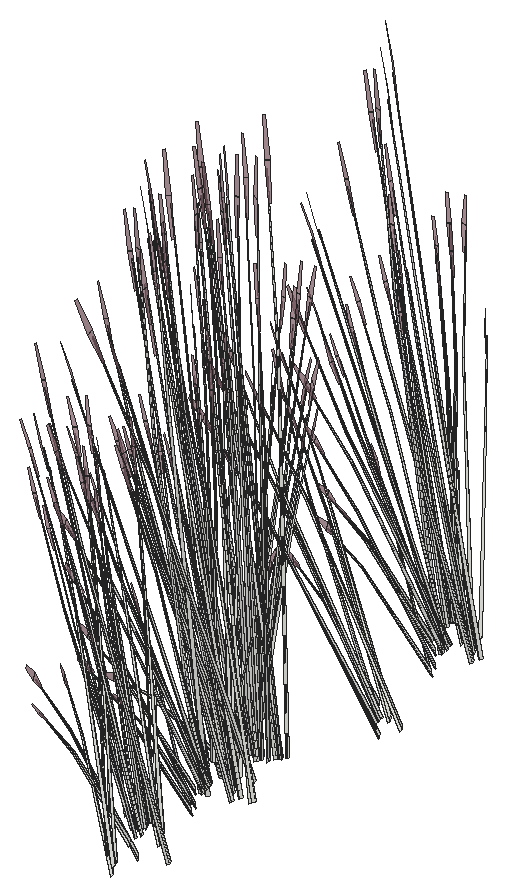
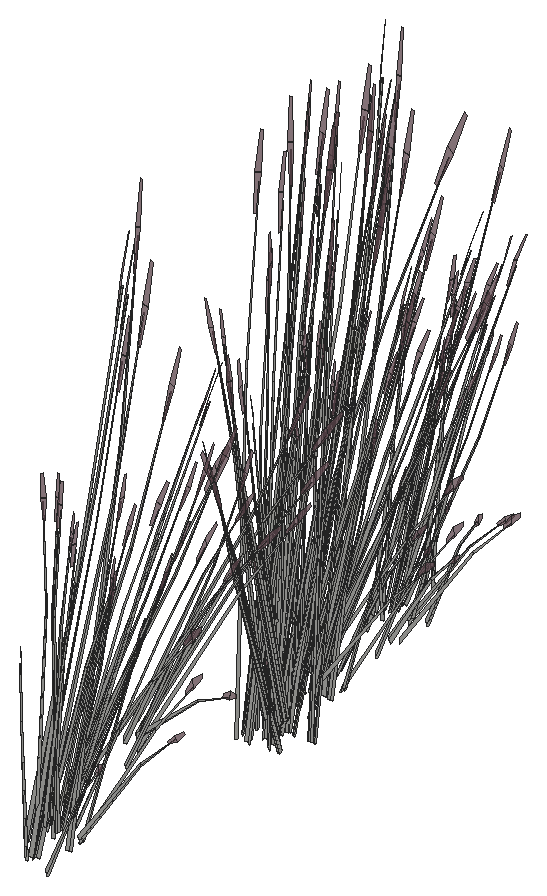
# SketchUp Ruby script. Lengths in inches.
U = 1.inch
M = Sketchup.active_model
def pt(a) = Geom::Point3d.new(a.map { |v| v * U })
def face(e, loops, mat)
  f = e.add_face(loops[0].map { |a| pt(a) })
  loops[1..].each { |l| e.add_face(l.map { |a| pt(a) }).erase! }
  f.material = f.back_material = mat if mat
  f
end
# faces: each face lists its corners as indices into pts; further lists are holes
def faces(e, pts, list, mat = nil) = list.each { |f| face(e, (f[0].is_a?(Array) ? f : [f]).map { |l| l.map { |i| pts[i] } }, mat) }
# xy, xz, yz: faces in a plane at the given z, y or x. An outline is a flat list of corners, or four numbers for a rectangle; further outlines are holes
def ring(l) = l.size == 4 ? [[l[0], l[1]], [l[2], l[1]], [l[2], l[3]], [l[0], l[3]]] : l.each_slice(2).to_a
def flat(e, list, mat, &to3) = list.each { |f| face(e, (f[0].is_a?(Array) ? f : [f]).map { |l| ring(l).map { |u, v| to3.(u, v) } }, mat) }
def xy(e, z, list, mat = nil) = flat(e, list, mat) { |x, y| [x, y, z] }
def xz(e, y, list, mat = nil) = flat(e, list, mat) { |x, z| [x, y, z] }
def yz(e, x, list, mat = nil) = flat(e, list, mat) { |y, z| [x, y, z] }
def lines(e, pts, list) = list.each { |a, b| e.add_line(pt(pts[a]), pt(pts[b])) }
# prism: a flat outline (further loops are holes) pulled along v
def prism(e, loops, v, mat = nil)
  f = face(e, loops, mat); d = Geom::Vector3d.new(v.map { |x| x * U })
  f.pushpull(f.normal.samedirection?(d) ? d.length : -d.length)
end
def box(e, o, s, mat = nil) = prism(e, [[o, [o[0] + s[0], o[1], o[2]], [o[0] + s[0], o[1] + s[1], o[2]], [o[0], o[1] + s[1], o[2]]]], [0, 0, s[2]], mat)
def at(x, y, z, deg = 0) = Geom::Transformation.translation(pt([x, y, z])) * Geom::Transformation.rotation(ORIGIN, Z_AXIS, deg.degrees)
def axes(o, x, y, z) = Geom::Transformation.new([*x, 0, *y, 0, *z, 0, *pt(o).to_a, 1])
def part(name) = M.definitions.add(name)
# library, detail: a bought-in or finely detailed component or shape, given as its bounding box
def library(name, o, s) = part(name).tap { |d| box(d.entities, o, s) }
def detail(e, o, s) = box(e.add_group.entities, o, s)
def put(e, d, t, mat = nil) = e.add_instance(d, t).tap { |i| i.material = mat if mat }
def group(e, t, mat = nil) = e.add_group.tap { |g| g.transformation = t; g.material = mat if mat }.entities
root = M.entities
M.materials.add("LightPink_Translucent").color = [144, 107, 117]
M.materials["LightPink_Translucent"].alpha = 0.75
c1 = part("blade")
p = [[2.15,0.21,22],[0,0.17,0],[0.09,0.45,0],[2.18,0.31,22],[2.29,0.31,22],[0.38,0.45,0],
  [2.48,0.24,33],[2.49,0.24,33],[2.48,0.22,33]]
faces(c1.entities,p,[[0,1,2,3],[4,5,2,3],[6,3,4,7],[8,0,3,6]])
c2 = part("seeds")
p = [[0.3,-0.1,1.38],[-0.01,-0.03,1.59],[-0.01,-0.03,0.03],[0.14,-0.07,-0.07],[0.29,-0.03,3],[0.15,0.01,3.11]]
faces(c2.entities,p,[[0,1,2,3],[1,0,4,5]],"LightPink_Translucent")
c3 = part("blade with seeds")
put(c3.entities,c1,at(0,0,0))
put(c3.entities,c2,axes([2.4,0.25,30.99],[1.5799,-0.05474,1.17369],[-0.12525,1.92788,0.29478],[-0.07173,-0.02425,1.56792]))
put(root,c3,axes([287.68,481.24,4.73],[-0.61415,-0.2744,0.0643],[0.35756,-0.39076,0.50621],[-0.1969,0.12633,0.77189]))
put(root,c3,axes([287.0625,487.16,2.21],[-0.53742,-0.54764,-0.44739],[0.81403,-0.38564,0.21531],[-0.17391,-0.06776,1.43643]))
put(root,c3,axes([288.45,511.57,4.73],[-0.32857,-0.44488,0.0643],[0.59916,-0.21775,0.50621],[-0.26412,0.04296,0.77189]))
put(root,c3,axes([289.96,512.8,3.875],[0.22344,-0.20048,1.71376],[0.56419,0.54113,0.13857],[-0.38697,0.24643,0.73262]))
put(root,c3,axes([288.62,513.33,4.53],[-0.77872,0.09325,-0.35414],[-0.20563,-0.53305,0.4572],[-0.22316,0.14318,0.87481]))
put(root,c3,axes([285.54,488.6,5.34],[-0.02328,0.60353,-0.7886],[-0.98022,-0.04053,0.09517],[-0.10344,0.25568,1.11556]))
put(root,c3,axes([285.52,490.3,2.77],[-0.02315,-0.38796,1.1486],[0.57853,0.27671,0.84392],[-0.11378,0.18492,0.25299]))
put(root,c3,axes([286.33,483.67,5.09],[0.99656,-0.1677,0.53763],[0.17295,0.65785,0.4433],[-0.23438,-0.19388,1.11249]))
put(root,c3,axes([290.03,468.16,4.53],[-0.74348,-0.18202,-0.35414],[0.21685,-0.53102,0.4572],[-0.29933,0.04869,0.87481]))
put(root,c3,axes([288.19,514.91,1.49],[0.12,0.06519,1.76342],[0.20347,0.60397,-0.26939],[-0.26596,0.12879,0.30037]))
put(root,c3,axes([288.93,481.44,3.875],[0.16657,-0.22426,1.71376],[0.69879,0.4641,0.13857],[-0.31524,0.28926,0.73262]))
put(root,c3,axes([288.21,487.55,2.21],[-0.97146,0.04028,-0.44739],[-0.08785,-0.66859,0.21531],[-0.17391,0.06776,1.43643]))
put(root,c3,axes([288.02,511.36,2.77],[0.57115,-0.04669,1.1486],[-0.36229,0.41137,0.84392],[-0.28224,-0.06171,0.25299]))
put(root,c3,axes([288.26,479.88,5.05],[0.74348,0.18202,0.35414],[-0.21685,0.53102,-0.4572],[-0.29933,0.04869,0.87481]))
put(root,c3,axes([286.5625,483.81,4.73],[0.4066,-0.41448,0.0643],[0.57901,0.24131,0.50621],[-0.18719,-0.13288,0.77189]))
put(root,c3,axes([288.72,513.21,4.73],[-0.22187,-0.60049,0.48003],[0.87033,-0.10422,0.3958],[-0.25651,0.14123,0.9933]))
put(root,c3,axes([287.9375,469.14,4.71],[0.11417,0.0175,1.77383],[0.35319,0.57649,-0.16761],[-0.23371,0.15131,0.31391]))
put(root,c3,axes([290.54,468.43,4.68],[-0.24236,0.59349,-0.51099],[-0.83094,-0.20343,-0.3958],[-0.33455,0.05442,0.97773]))
put(root,c3,axes([286.35,488.67,2.48],[0.83726,0.32623,0.49651],[-0.50045,0.58498,0],[-0.19069,-0.0743,1.57504]))
put(root,c3,axes([288.39,481.53,4.68],[0.22982,0.59576,-0.51099],[-0.87033,0.10422,-0.3958],[-0.24941,0.16002,0.97773]))
put(root,c3,axes([285.21,489.45,3.36],[0.01966,-0.33682,1.54345],[0.88405,0.17791,0.21329],[-0.0766,0.35897,0.72882]))
put(root,c3,axes([289.17,510.22,5.09],[0.7388,-0.48151,0.53763],[0.63717,0.51135,0.4433],[-0.34662,-0.08882,1.11249]))
put(root,c3,axes([288.64,478.36,4.73],[0.04505,-0.49615,0.0643],[0.68022,0.0136,0.50621],[-0.26056,-0.05192,0.77189]))
put(root,c3,axes([287.03,482.6,4.72],[-0.02224,0.12912,1.74944],[0.63107,0.44917,-0.27667],[-0.16521,0.21241,0.14031]))
put(root,c3,axes([287.14,487.47,2.4375],[0.23711,-0.77313,-0.23429],[1.12425,0.13477,0.51271],[-0.19645,-0.10677,1.5644]))
put(root,c3,axes([288.54,513.1,4.73],[-0.61415,-0.2744,0.0643],[0.35756,-0.39076,0.50621],[-0.1969,0.12633,0.77189]))
put(root,c3,axes([290.12,468.39,1.49],[0.02269,0.10283,1.76342],[-0.45738,0.53699,-0.26939],[-0.32488,-0.02707,0.30037]))
put(root,c3,axes([290.5625,481.11,2.06],[-0.9306,-0.10697,-0.62353],[0.19638,-0.65984,-0.16365],[-0.27771,-0.07995,1.37633]))
put(root,c3,axes([290.73,477.51,5.43],[-0.59706,0.6255,-0.13619],[-0.86465,-0.36036,-0.75594],[-0.30056,-0.17672,1.14864]))
put(root,c3,axes([287.55,487.65,2.62],[-0.17258,0.58229,0.1448],[-0.84319,-0.10108,-0.41347],[-0.15345,-0.05979,1.26744]))
put(root,c3,axes([289.1,478.74,5.05],[0.50902,0.40851,0.35414],[-0.58122,0.38671,-0.4572],[-0.29531,-0.05884,0.87481]))
put(root,c3,axes([287.45,482.58,4.72],[-0.13683,-0.09148,1.74944],[-0.91315,0.058,-0.27667],[-0.14574,-0.2188,0.14031]))
put(root,c3,axes([289.23,489.27,2.02],[-0.83726,0.32623,-0.49651],[-0.50045,-0.58498,0],[-0.19069,0.0743,1.57504]))
put(root,c3,axes([289.79,513.3,3.875],[0.16657,-0.22426,1.71376],[0.69879,0.4641,0.13857],[-0.31524,0.28926,0.73262]))
put(root,c3,axes([284.27,486.02,2.02],[0,-0.65246,-0.49651],[1.00089,0,0],[0,-0.1486,1.57504]))
put(root,c3,axes([290.47,478.01,4.98],[-0.76283,-0.31537,-0.71045],[0.54213,-0.55263,0.08574],[-0.27638,-0.1883,1.00501]))
put(root,c3,axes([284.7,486.63,2.48],[0,0.65246,0.49651],[-1.00089,0,0],[0,-0.1486,1.57504]))
put(root,c3,axes([289.28,489.1,2.19],[-0.55235,-0.65609,-0.05142],[0.93577,-0.36461,0.51607],[-0.23059,0.06247,1.6363]))
put(root,c3,axes([290.11,478.03,4.68],[-0.88277,0.1551,-0.51099],[-0.15442,-0.58737,-0.3958],[-0.23711,-0.16832,0.97773]))
put(root,c3,axes([288.89,470.97,2.77],[0.37283,-0.29571,1.1486],[0.14711,0.46813,0.84392],[-0.26943,0.08382,0.25299]))
put(root,c3,axes([293.77,496.78,3.875],[0.37107,-0.01478,1.71376],[-0.24616,0.64047,0.13857],[-0.5288,-0.03961,0.73262]))
put(root,c3,axes([289.125,511.74,5.05],[0.74348,0.18202,0.35414],[-0.21685,0.53102,-0.4572],[-0.29933,0.04869,0.87481]))
put(root,c3,axes([285.74,488.8,5],[0.64041,0.4384,-0.5672],[-0.67652,0.38394,-0.43934],[-0.09744,0.22274,1.08528]))
put(root,c3,axes([289.34,482.35,2.02],[-0.83726,-0.32623,-0.49651],[0.50045,-0.58498,0],[-0.19069,-0.0743,1.57504]))
put(root,c3,axes([290.2,468.09,4.73],[0.25275,-0.59491,0.48003],[0.83094,0.20343,0.3958],[-0.32677,0.03575,0.9933]))
put(root,c3,axes([289.03,489.02,2.03],[-0.83462,-0.16144,-0.30978],[0.21015,-0.56852,0.30978],[-0.16826,0.06556,1.38974]))
put(root,c3,axes([288.98,477.49,1.49],[-0.08666,0.08595,1.76342],[-0.87574,0.18531,-0.26939],[-0.21156,-0.16858,0.30037]))
put(root,c3,axes([287.98,481.11,5.03],[0.82753,0.35977,-0.1216],[-0.47675,0.52101,-0.67495],[-0.2338,0.18111,1.02557]))
put(root,c3,axes([285.45,488.48,5.05],[0.60531,-0.34352,0.35414],[0.573,0.39225,-0.4572],[-0.08718,0.19929,0.87481]))
put(root,c3,axes([290.5,467.92,5.03],[0.45012,0.59081,-0.1216],[-0.79888,0.29033,-0.67495],[-0.33665,0.07795,1.02557]))
put(root,c3,axes([289.26,513.39,4.68],[0.22982,0.59576,-0.51099],[-0.87033,0.10422,-0.3958],[-0.24941,0.16002,0.97773]))
put(root,c3,axes([291.51,466.69,5.03],[-0.0479,0.66354,-0.1216],[-0.90696,-0.01814,-0.67495],[-0.3493,-0.04609,1.02557]))
put(root,c3,axes([286.89,486.78,2.67],[-1.00749,-0.31132,-0.29095],[0.48511,-0.65709,-0.50002],[-0.03166,-0.16133,1.59708]))
put(root,c3,axes([289.51,486.59,2.84],[-0.02444,-0.61432,1.41272],[1.10603,0.15924,0.59816],[-0.26159,0.33615,1.3335]))
put(root,c3,axes([289.5,510.22,4.73],[0.04505,-0.49615,0.0643],[0.68022,0.0136,0.50621],[-0.26056,-0.05192,0.77189]))
put(root,c3,axes([289.85,482.75,2.375],[-0.55932,0.6538,0],[-0.93577,-0.36461,-0.51607],[-0.21313,-0.08304,1.63711]))
put(root,c3,axes([290.14,467.94,4.73],[-0.32857,-0.44488,0.0643],[0.59916,-0.21775,0.50621],[-0.26412,0.04296,0.77189]))
put(root,c3,axes([287.9,514.46,4.72],[-0.02224,0.12912,1.74944],[0.63107,0.44917,-0.27667],[-0.16521,0.21241,0.14031]))
put(root,c3,axes([291.64,469.17,3.875],[0.22344,-0.20048,1.71376],[0.56419,0.54113,0.13857],[-0.38697,0.24643,0.73262]))
put(root,c3,axes([290.3,469.69,4.53],[-0.77872,0.09325,-0.35414],[-0.20563,-0.53305,0.4572],[-0.22316,0.14318,0.87481]))
put(root,c3,axes([291.43,512.96,2.06],[-0.9306,-0.10697,-0.62353],[0.19638,-0.65984,-0.16365],[-0.27771,-0.07995,1.37633]))
put(root,c3,axes([291.6,509.36,5.43],[-0.59706,0.6255,-0.13619],[-0.86465,-0.36036,-0.75594],[-0.30056,-0.17672,1.14864]))
put(root,c3,axes([291.74,462.66,3.875],[0.22344,-0.20048,1.71376],[0.56419,0.54113,0.13857],[-0.38697,0.24643,0.73262]))
put(root,c3,axes([289.96,510.59,5.05],[0.50902,0.40851,0.35414],[-0.58122,0.38671,-0.4572],[-0.29531,-0.05884,0.87481]))
put(root,c3,axes([285.07,488.57,5.4],[0.98321,0.03233,-0.13498],[-0.02687,0.61208,-0.74919],[-0.0683,0.23574,1.13838]))
put(root,c3,axes([289.875,471.27,1.49],[0.12,0.06519,1.76342],[0.20347,0.60397,-0.26939],[-0.26596,0.12879,0.30037]))
put(root,c3,axes([285.04,489.46,2.82],[0.8127,-0.11554,0.06507],[0.18684,0.46549,-0.86304],[-0.05152,0.23564,0.7736]))
put(root,c3,axes([291.33,509.87,4.98],[-0.76283,-0.31537,-0.71045],[0.54213,-0.55263,0.08574],[-0.27638,-0.1883,1.00501]))
put(root,c3,axes([289.7,467.72,2.77],[0.57115,-0.04669,1.1486],[-0.36229,0.41137,0.84392],[-0.28224,-0.06171,0.25299]))
put(root,c3,axes([288.89,487.37,2.67],[0.10425,0.7445,-0.29095],[-1.08575,0.04502,-0.50002],[-0.19119,0.09917,1.59708]))
put(root,c3,axes([286.62,482.67,5.65],[0.78943,0.17416,-0.06488],[-0.24284,0.53604,-0.29416],[-0.12912,0.08139,0.97024]))
put(root,c3,axes([289.97,464.77,1.49],[0.12,0.06519,1.76342],[0.20347,0.60397,-0.26939],[-0.26596,0.12879,0.30037]))
put(root,c3,axes([290.98,509.89,4.68],[-0.88277,0.1551,-0.51099],[-0.15442,-0.58737,-0.3958],[-0.23711,-0.16832,0.97773]))
put(root,c3,axes([286.44,486.12,2.1],[-0.36739,-0.66907,-0.69835],[1.05831,-0.24096,-0.18329],[-0.04061,-0.22656,1.54149]))
put(root,c3,axes([288.84,483.99,5.03],[-0.87543,0.30377,-0.1216],[-0.4302,-0.53915,-0.67495],[-0.1155,-0.2272,1.02557]))
put(root,c3,axes([288.09,484.02,4.68],[-0.87941,-0.16356,-0.51099],[0.30143,-0.56078,-0.3958],[-0.08064,-0.22578,0.97773]))
put(root,c3,axes([288.39,481.16,5.05],[0.77872,-0.09325,0.35414],[0.20563,0.53305,-0.4572],[-0.22316,0.14318,0.87481]))
put(root,c3,axes([286.47,488.17,3.875],[-0.0219,-0.25042,1.71376],[0.94901,0.16613,0.13857],[-0.0587,0.35688,0.73262]))
put(root,c3,axes([293.92,497.91,3.875],[0.31041,-0.13801,1.71376],[0.26133,0.63772,0.13857],[-0.48731,0.14413,0.73262]))
put(root,c3,axes([290.4,469.57,4.73],[-0.22187,-0.60049,0.48003],[0.87033,-0.10422,0.3958],[-0.25651,0.14123,0.9933]))
put(root,c3,axes([288.83,483.69,2.59],[0.28231,-0.10293,1.43002],[0.69701,0.31035,-0.30754],[-0.20746,0.26854,0.61141]))
put(root,c3,axes([290.21,514.21,2.02],[-0.83726,-0.32623,-0.49651],[0.50045,-0.58498,0],[-0.19069,-0.0743,1.57504]))
put(root,c3,axes([289.84,509.35,1.49],[-0.08666,0.08595,1.76342],[-0.87574,0.18531,-0.26939],[-0.21156,-0.16858,0.30037]))
put(root,c3,axes([288.85,512.96,5.03],[0.82753,0.35977,-0.1216],[-0.47675,0.52101,-0.67495],[-0.2338,0.18111,1.02557]))
put(root,c3,axes([288.43,477.83,2.13],[-0.25807,0.53277,-0.03893],[-0.79428,-0.16389,-0.17649],[-0.1206,-0.08714,0.58215]))
put(root,c3,axes([284.7,486.04,2.03],[0.62448,-0.40708,-0.30978],[0.62448,0.40708,0.30978],[0,-0.13112,1.38974]))
put(root,c3,axes([287.52,483.41,2.13],[-0.61821,0.37431,-0.03893],[-0.56645,-0.40995,-0.17649],[-0.03988,-0.11616,0.58215]))
put(root,c3,axes([292.96,498.99,2.59],[0.3109,0.05356,1.43002],[0.20038,0.54709,-0.30754],[-0.42231,0.10241,0.61141]))
put(root,c3,axes([290.23,469.46,4.73],[-0.61415,-0.2744,0.0643],[0.35756,-0.39076,0.50621],[-0.1969,0.12633,0.77189]))
put(root,c3,axes([290.72,514.6,2.375],[-0.55932,0.6538,0],[-0.93577,-0.36461,-0.51607],[-0.21313,-0.08304,1.63711]))
put(root,c3,axes([287.27,487.1,2.36],[1.13071,0.13747,0.45755],[-0.23011,0.77639,0.17955],[-0.16524,-0.07497,1.58856]))
put(root,c3,axes([290.5,476.02,4.71],[-0.01669,0.07821,1.77383],[-0.82314,0.28383,-0.16761],[-0.24223,-0.14508,0.31391]))
put(root,c3,axes([289.62,477.15,2.59],[-0.05417,0.21344,1.43002],[-0.79196,0.17867,-0.30754],[-0.18512,-0.27588,0.61141]))
put(root,c3,axes([289.875,477.71,3.875],[0.2045,0.20949,1.71376],[-0.94495,0.17636,0.13857],[-0.21357,-0.32887,0.73262]))
put(root,c3,axes([295.71,497.24,3.34],[0.25429,-0.09438,1.77064],[0.08769,0.65901,0.13857],[-0.5508,0.08745,0.63284]))
put(root,c3,axes([291.48,469.66,3.875],[0.16657,-0.22426,1.71376],[0.69879,0.4641,0.13857],[-0.31524,0.28926,0.73262]))
put(root,c3,axes([291.62,481.2,2.67],[-0.90324,0.43318,-0.29095],[-0.60064,-0.61207,-0.50002],[-0.22285,-0.06216,1.59708]))
put(root,c3,axes([286.98,486.96,2.72],[-0.43405,0.58792,0.44739],[-0.90188,-0.28295,-0.21531],[0,-0.13553,1.43643]))
put(root,c3,axes([288.41,484.125,4.98],[-0.42698,-0.53052,-0.71045],[0.87893,-0.29566,0.08574],[-0.09984,-0.25633,1.00501]))
put(root,c3,axes([289.125,482.57,4.73],[-0.63704,-0.44518,0.48003],[0.67652,-0.38394,0.3958],[-0.11751,0.20886,0.9933]))
put(root,c3,axes([287.48,514.53,5.65],[0.78943,0.17416,-0.06488],[-0.24284,0.53604,-0.29416],[-0.12912,0.08139,0.97024]))
put(root,c3,axes([291.58,463.15,3.875],[0.16657,-0.22426,1.71376],[0.69879,0.4641,0.13857],[-0.31524,0.28926,0.73262]))
put(root,c3,axes([290.21,477.6,4.53],[-0.13817,-0.52554,-0.35414],[0.78985,-0.13877,0.4572],[-0.21215,-0.1506,0.87481]))
put(root,c3,axes([289.25,513.01,5.05],[0.77872,-0.09325,0.35414],[0.20563,0.53305,-0.4572],[-0.22316,0.14318,0.87481]))
put(root,c3,axes([288,480.26,2.375],[-1.11865,0,0],[0,-0.72922,-0.51607],[0,-0.16609,1.63711]))
put(root,c3,axes([289.58,482.11,2.03],[-0.21015,-0.56852,-0.30978],[0.83462,-0.16144,0.30978],[-0.16826,-0.06556,1.38974]))
put(root,c3,axes([290.8125,468.1,5.05],[0.74348,0.18202,0.35414],[-0.21685,0.53102,-0.4572],[-0.29933,0.04869,0.87481]))
put(root,c3,axes([288.89,482.53,4.73],[-0.73517,-0.0304,0.0643],[0.02016,-0.45906,0.50621],[-0.07693,0.17585,0.77189]))
put(root,c3,axes([289.7,515.55,2.59],[0.28231,-0.10293,1.43002],[0.69701,0.31035,-0.30754],[-0.20746,0.26854,0.61141]))
put(root,c3,axes([286.66,488.34,2.47],[0.96132,-0.17317,0.17642],[0.23737,0.64447,0.35086],[-0.08574,-0.0939,1.60407]))
put(root,c3,axes([289.12,482.7,4.53],[-0.60531,0.34352,-0.35414],[-0.573,-0.39225,0.4572],[-0.08718,0.19929,0.87481]))
put(root,c3,axes([289.3,509.68,2.13],[-0.25807,0.53277,-0.03893],[-0.79428,-0.16389,-0.17649],[-0.1206,-0.08714,0.58215]))
put(root,c3,axes([290.94,469.75,4.68],[0.22982,0.59576,-0.51099],[-0.87033,0.10422,-0.3958],[-0.24941,0.16002,0.97773]))
put(root,c3,axes([291.04,463.25,4.68],[0.22982,0.59576,-0.51099],[-0.87033,0.10422,-0.3958],[-0.24941,0.16002,0.97773]))
put(root,c3,axes([287.9,488.44,2.2],[-0.90188,-0.29293,0],[0.43405,-0.60866,0],[0,0,1.62707]))
put(root,c3,axes([289.58,470.82,4.72],[-0.02224,0.12912,1.74944],[0.63107,0.44917,-0.27667],[-0.16521,0.21241,0.14031]))
put(root,c3,axes([292.97,497.68,4.72],[-0.14609,0.08471,1.74944],[0.01243,0.61893,-0.27667],[-0.33486,0.08049,0.14031]))
put(root,c3,axes([288.58,484.2,5.05],[-0.2697,0.50175,0.35414],[-0.78684,-0.14635,-0.4572],[-0.07215,-0.20201,0.87481]))
put(root,c3,axes([289.99,489.17,2.375],[0.55932,0.6538,0],[-0.93577,0.36461,-0.51607],[-0.21313,0.08304,1.63711]))
put(root,c3,axes([294.88,496.19,4.98],[-0.89428,-0.01571,-0.71045],[0.06006,-0.66153,0.08574],[-0.37886,-0.06981,1.00501]))
put(root,c3,axes([293.11,469.32,2.06],[-0.9306,-0.10697,-0.62353],[0.19638,-0.65984,-0.16365],[-0.27771,-0.07995,1.37633]))
put(root,c3,axes([291.36,507.875,4.71],[-0.01669,0.07821,1.77383],[-0.82314,0.28383,-0.16761],[-0.24223,-0.14508,0.31391]))
put(root,c3,axes([289.68,464.32,4.72],[-0.02224,0.12912,1.74944],[0.63107,0.44917,-0.27667],[-0.16521,0.21241,0.14031]))
put(root,c3,axes([292.22,481.68,2.06],[-0.60257,0.49041,-0.62353],[-0.74854,-0.44469,-0.16365],[-0.24146,0.12234,1.37633]))
put(root,c3,axes([294.16,496.35,2.59],[0.17466,0.18165,1.43002],[-0.40248,0.49377,-0.30754],[-0.41327,-0.11802,0.61141]))
put(root,c3,axes([290.67,478.03,5.05],[0.13817,0.52554,0.35414],[-0.78985,0.13877,-0.4572],[-0.21215,-0.1506,0.87481]))
put(root,c3,axes([290.48,509.01,2.59],[-0.05417,0.21344,1.43002],[-0.79196,0.17867,-0.30754],[-0.18512,-0.27588,0.61141]))
put(root,c3,axes([287.14,489.46,5.0625],[-0.88151,-0.17057,0.53283],[0.30143,-0.56078,0.43934],[0.05297,0.22053,1.10256]))
put(root,c3,axes([291.65,466.95,5.05],[0.50902,0.40851,0.35414],[-0.58122,0.38671,-0.4572],[-0.29531,-0.05884,0.87481]))
put(root,c3,axes([286.96,483.93,4.71],[0.10149,-0.03939,1.77383],[0.83886,0.26202,-0.16761],[-0.01971,0.21816,0.31391]))
put(root,c3,axes([288.87,480.07,2.33],[-0.83213,0.54855,0.30756],[-0.83263,-0.54278,-0.36492],[-0.02906,-0.15578,1.64885]))
put(root,c3,axes([290.74,509.5625,3.875],[0.2045,0.20949,1.71376],[-0.94495,0.17636,0.13857],[-0.21357,-0.32887,0.73262]))
put(root,c3,axes([293.44,497.33,4.53],[-0.74348,-0.18202,-0.35414],[0.21685,-0.53102,0.4572],[-0.29933,0.04869,0.87481]))
put(root,c3,axes([292.48,513.06,2.67],[-0.90324,0.43318,-0.29095],[-0.60064,-0.61207,-0.50002],[-0.22285,-0.06216,1.59708]))
put(root,c3,axes([286.91,489.5,4.73],[-0.6592,0.22175,0.0643],[-0.32265,-0.40436,0.50621],[0.06366,0.17825,0.77189]))
put(root,c3,axes([294.47,495.75,3.875],[0.3323,0.11241,1.71376],[-0.68769,0.4716,0.13857],[-0.42861,-0.21275,0.73262]))
put(root,c3,axes([289.99,514.43,4.73],[-0.63704,-0.44518,0.48003],[0.67652,-0.38394,0.3958],[-0.11751,0.20886,0.9933]))
put(root,c3,axes([292.3,481.58,3.33],[0.77308,0.2631,1.51261],[-0.75736,0.56681,0.59816],[-0.33924,-0.33594,1.26806]))
put(root,c3,axes([289.52,488.375,2.47],[0.25843,-0.64844,0.17642],[0.9457,0.1835,0.35086],[-0.16336,0.00316,1.60407]))
put(root,c3,axes([289.09,487.51,2.62],[0.66093,0.39201,0.1448],[-0.5513,0.44227,-0.41347],[-0.15345,0.05979,1.26744]))
put(root,c3,axes([291.07,509.45,4.53],[-0.13817,-0.52554,-0.35414],[0.78985,-0.13877,0.4572],[-0.21215,-0.1506,0.87481]))
put(root,c3,axes([289.35,476.81,2.77],[0.46666,0.22709,1.1486],[-0.67962,0.13651,0.84392],[-0.14541,-0.17452,0.25299]))
put(root,c3,axes([288.87,512.11,2.375],[-1.11865,0,0],[0,-0.72922,-0.51607],[0,-0.16609,1.63711]))
put(root,c3,axes([290.44,513.97,2.03],[-0.21015,-0.56852,-0.30978],[0.83462,-0.16144,0.30978],[-0.16826,-0.06556,1.38974]))
put(root,c3,axes([292.63,481.4,2.46],[-0.87356,-0.52515,-0.25192],[0.73507,-0.5897,0.5513],[-0.23523,0.06143,1.68216]))
